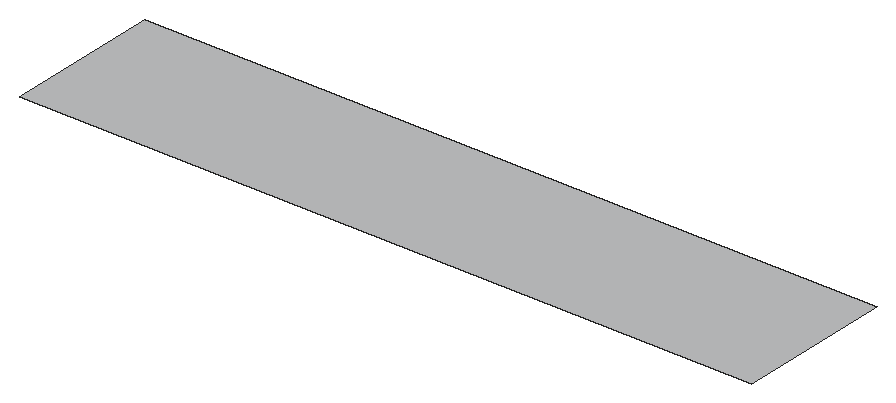
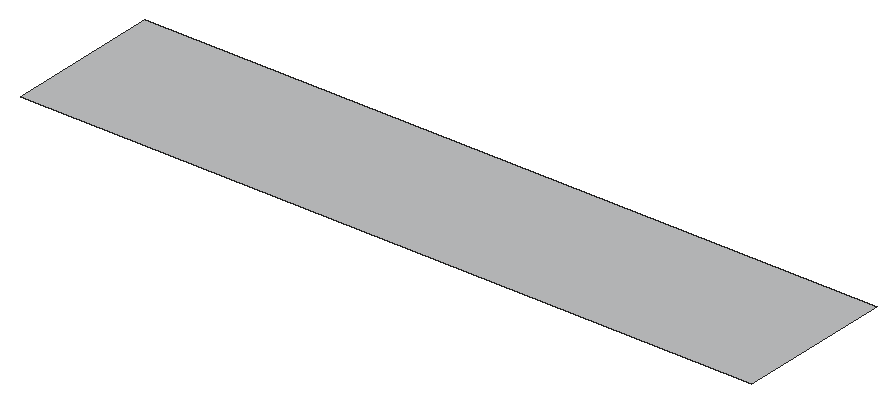
# SketchUp Ruby script. Lengths in inches.
U = 1.inch
M = Sketchup.active_model
def pt(a) = Geom::Point3d.new(a.map { |v| v * U })
def face(e, loops, mat)
  f = e.add_face(loops[0].map { |a| pt(a) })
  loops[1..].each { |l| e.add_face(l.map { |a| pt(a) }).erase! }
  f.material = f.back_material = mat if mat
  f
end
# faces: each face lists its corners as indices into pts; further lists are holes
def faces(e, pts, list, mat = nil) = list.each { |f| face(e, (f[0].is_a?(Array) ? f : [f]).map { |l| l.map { |i| pts[i] } }, mat) }
# xy, xz, yz: faces in a plane at the given z, y or x. An outline is a flat list of corners, or four numbers for a rectangle; further outlines are holes
def ring(l) = l.size == 4 ? [[l[0], l[1]], [l[2], l[1]], [l[2], l[3]], [l[0], l[3]]] : l.each_slice(2).to_a
def flat(e, list, mat, &to3) = list.each { |f| face(e, (f[0].is_a?(Array) ? f : [f]).map { |l| ring(l).map { |u, v| to3.(u, v) } }, mat) }
def xy(e, z, list, mat = nil) = flat(e, list, mat) { |x, y| [x, y, z] }
def xz(e, y, list, mat = nil) = flat(e, list, mat) { |x, z| [x, y, z] }
def yz(e, x, list, mat = nil) = flat(e, list, mat) { |y, z| [x, y, z] }
def lines(e, pts, list) = list.each { |a, b| e.add_line(pt(pts[a]), pt(pts[b])) }
# prism: a flat outline (further loops are holes) pulled along v
def prism(e, loops, v, mat = nil)
  f = face(e, loops, mat); d = Geom::Vector3d.new(v.map { |x| x * U })
  f.pushpull(f.normal.samedirection?(d) ? d.length : -d.length)
end
def box(e, o, s, mat = nil) = prism(e, [[o, [o[0] + s[0], o[1], o[2]], [o[0] + s[0], o[1] + s[1], o[2]], [o[0], o[1] + s[1], o[2]]]], [0, 0, s[2]], mat)
def at(x, y, z, deg = 0) = Geom::Transformation.translation(pt([x, y, z])) * Geom::Transformation.rotation(ORIGIN, Z_AXIS, deg.degrees)
def axes(o, x, y, z) = Geom::Transformation.new([*x, 0, *y, 0, *z, 0, *pt(o).to_a, 1])
def part(name) = M.definitions.add(name)
# library, detail: a bought-in or finely detailed component or shape, given as its bounding box
def library(name, o, s) = part(name).tap { |d| box(d.entities, o, s) }
def detail(e, o, s) = box(e.add_group.entities, o, s)
def put(e, d, t, mat = nil) = e.add_instance(d, t).tap { |i| i.material = mat if mat }
def group(e, t, mat = nil) = e.add_group.tap { |g| g.transformation = t; g.material = mat if mat }.entities
root = M.entities
M.materials.add("[Fencing Metal Straight]").color = [194, 195, 196]
xy(root,115.1875,[[14.48,0,113.3,21.02]],"[Fencing Metal Straight]")
